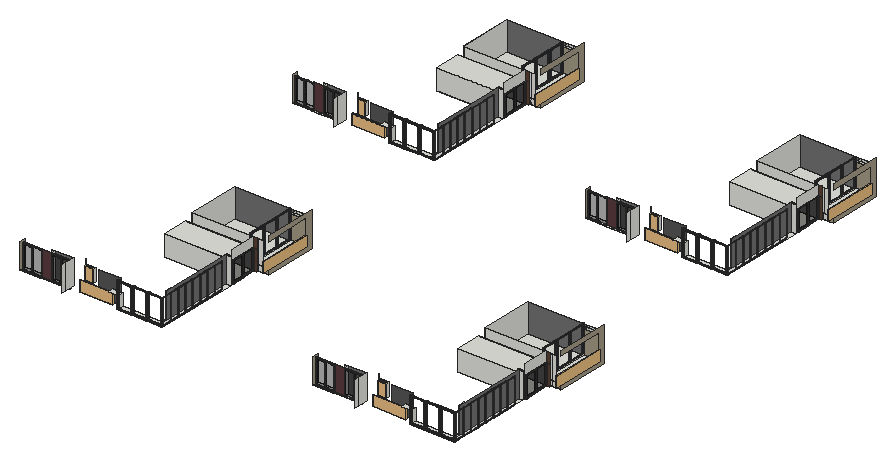
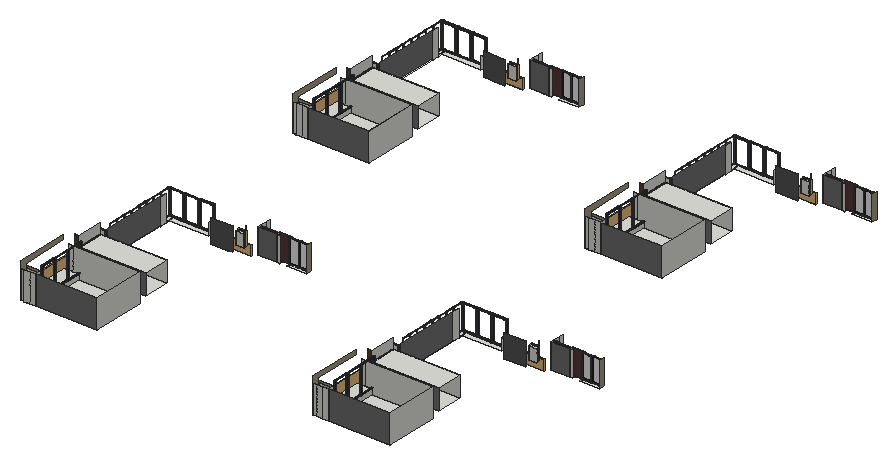
# SketchUp Ruby script. Lengths in inches.
U = 1.inch
M = Sketchup.active_model
def pt(a) = Geom::Point3d.new(a.map { |v| v * U })
def face(e, loops, mat)
  f = e.add_face(loops[0].map { |a| pt(a) })
  loops[1..].each { |l| e.add_face(l.map { |a| pt(a) }).erase! }
  f.material = f.back_material = mat if mat
  f
end
# faces: each face lists its corners as indices into pts; further lists are holes
def faces(e, pts, list, mat = nil) = list.each { |f| face(e, (f[0].is_a?(Array) ? f : [f]).map { |l| l.map { |i| pts[i] } }, mat) }
# xy, xz, yz: faces in a plane at the given z, y or x. An outline is a flat list of corners, or four numbers for a rectangle; further outlines are holes
def ring(l) = l.size == 4 ? [[l[0], l[1]], [l[2], l[1]], [l[2], l[3]], [l[0], l[3]]] : l.each_slice(2).to_a
def flat(e, list, mat, &to3) = list.each { |f| face(e, (f[0].is_a?(Array) ? f : [f]).map { |l| ring(l).map { |u, v| to3.(u, v) } }, mat) }
def xy(e, z, list, mat = nil) = flat(e, list, mat) { |x, y| [x, y, z] }
def xz(e, y, list, mat = nil) = flat(e, list, mat) { |x, z| [x, y, z] }
def yz(e, x, list, mat = nil) = flat(e, list, mat) { |y, z| [x, y, z] }
def lines(e, pts, list) = list.each { |a, b| e.add_line(pt(pts[a]), pt(pts[b])) }
# prism: a flat outline (further loops are holes) pulled along v
def prism(e, loops, v, mat = nil)
  f = face(e, loops, mat); d = Geom::Vector3d.new(v.map { |x| x * U })
  f.pushpull(f.normal.samedirection?(d) ? d.length : -d.length)
end
def box(e, o, s, mat = nil) = prism(e, [[o, [o[0] + s[0], o[1], o[2]], [o[0] + s[0], o[1] + s[1], o[2]], [o[0], o[1] + s[1], o[2]]]], [0, 0, s[2]], mat)
def at(x, y, z, deg = 0) = Geom::Transformation.translation(pt([x, y, z])) * Geom::Transformation.rotation(ORIGIN, Z_AXIS, deg.degrees)
def axes(o, x, y, z) = Geom::Transformation.new([*x, 0, *y, 0, *z, 0, *pt(o).to_a, 1])
def part(name) = M.definitions.add(name)
# library, detail: a bought-in or finely detailed component or shape, given as its bounding box
def library(name, o, s) = part(name).tap { |d| box(d.entities, o, s) }
def detail(e, o, s) = box(e.add_group.entities, o, s)
def put(e, d, t, mat = nil) = e.add_instance(d, t).tap { |i| i.material = mat if mat }
def group(e, t, mat = nil) = e.add_group.tap { |g| g.transformation = t; g.material = mat if mat }.entities
root = M.entities
M.materials.add("Glass_Tinted_Gray").color = [0, 0, 0]
M.materials["Glass_Tinted_Gray"].alpha = 0.125
M.materials.add("Glazing").color = [128, 128, 128]
M.materials["Glazing"].alpha = 0.05
M.materials.add("Powdercoating").color = [41, 44, 40]
M.materials.add("Wine2").color = [0, 0, 0]
M.materials["Wine2"].alpha = 0
M.materials.add("[0130_Gainsboro]").color = [39, 45, 50]
M.materials.add("[0135_DarkGray]").color = [81, 81, 81]
M.materials.add("[Color M05]").color = [114, 114, 114]
M.materials.add("[Color M06]").color = [86, 86, 86]
M.materials.add("[Concrete Tile]").color = [165, 155, 133]
M.materials.add("[Granite Brown]").color = [89, 59, 61]
M.materials.add("[Granite Brown]1").color = [89, 63, 50]
M.materials.add("[Mirror 02]").color = [229, 229, 229]
M.materials.add("[Terrazzo Light Blue]").color = [196, 214, 227]
c1 = library("Glass Railing",[0,0,0],[139.5,4.76,42])
c2 = part("PENTEK_RP Fineline 50S_Sliding_DoorCase_E1")
box(c2.entities,[0,0,0],[1.51,3.66,99.27],"[0135_DarkGray]")
c3 = part("PENTEK_RP Fineline 50S_SlidingDooe_Case_E2")
box(c3.entities,[0,0,0],[96.25,3.66,1.51],"[0135_DarkGray]")
c4 = part("pentek_RP Fineline 50S_SlidingDoor_Case")
put(c4.entities,c2,at(97.76,0,0))
put(c4.entities,c3,at(1.51,0,0))
put(c4.entities,c2,at(0,0,0))
put(c4.entities,c3,at(1.51,0,97.76))
c5 = part("PENTEK_RP Fineline 50S_SlidingDoor_GlazingBead_2")
box(c5.entities,[0,0,0],[0.56,0.59,94.39],"[0135_DarkGray]")
c6 = part("PENTEK_RP Fineline 50S_SlidingDoor_Glass")
box(c6.entities,[0,0,0],[46.58,0.16,94.39],"Glass_Tinted_Gray")
c7 = part("PENTEK_RP Fineline 50S_SlidingDoor_GlazingBead")
box(c7.entities,[0,0,0],[45.47,0.59,0.56],"[0135_DarkGray]")
c8 = part("PENTEK_RP Fineline 50S_SlidingDoor_Leaf_E1")
xy(c8.entities,0,[[0,0,0.93,1.97],[0.93,1.57,1.49,1.97]],"[0135_DarkGray]")
xy(c8.entities,96.25,[[0,0,0.93,0,0.93,1.57,1.49,1.57,1.49,1.97,0,1.97]],"[0135_DarkGray]")
xz(c8.entities,0,[[0,0,0.93,96.25]],"[0135_DarkGray]")
xz(c8.entities,1.57,[[0.93,0,1.49,95.32],[0.93,95.32,1.49,96.25]],"[0135_DarkGray]")
xz(c8.entities,1.97,[[0,0,1.49,96.25]],"[0135_DarkGray]")
yz(c8.entities,0,[[0,0,1.97,96.25]],"[0135_DarkGray]")
yz(c8.entities,0.93,[[0,0,1.57,0.93],[0,0.93,1.57,95.32],[0,95.32,1.57,96.25]],"[0135_DarkGray]")
yz(c8.entities,1.49,[[1.57,0,1.97,95.32],[1.57,95.32,1.97,96.25]],"[0135_DarkGray]")
c9 = part("PENTEK_RP Fineline 50S_SlidingDoor_Leaf_E2")
xy(c9.entities,0,[[0,0,0,1.57,0.56,1.57,0.56,1.97,46.02,1.97,46.02,1.57,46.58,1.57,46.58,0]],"[0135_DarkGray]")
xy(c9.entities,0.93,[[0,0,46.58,1.57]],"[0135_DarkGray]")
xy(c9.entities,1.49,[[0.56,1.57,46.02,1.97]],"[0135_DarkGray]")
xz(c9.entities,0,[[0,0,46.58,0.93]],"[0135_DarkGray]")
xz(c9.entities,1.57,[[0,0,0.56,0.93],[46.02,0,46.58,0.93],[0.56,0.93,46.02,1.49]],"[0135_DarkGray]")
xz(c9.entities,1.97,[[0.56,0,46.02,1.49]],"[0135_DarkGray]")
yz(c9.entities,0,[[0,0,1.57,0.93]],"[0135_DarkGray]")
yz(c9.entities,0.56,[[1.57,0,1.97,0.93],[1.57,0.93,1.97,1.49]],"[0135_DarkGray]")
yz(c9.entities,46.02,[[1.57,0,1.97,0.93],[1.57,0.93,1.97,1.49]],"[0135_DarkGray]")
yz(c9.entities,46.58,[[0,0,1.57,0.93]],"[0135_DarkGray]")
c10 = part("PENTEK_RP Fineline S_SlidingDoor_Leaf1")
put(c10.entities,c5,at(0.93,0,0.93))
put(c10.entities,c5,at(46.96,0,0.93))
put(c10.entities,c6,at(1.49,1.42,0.93))
put(c10.entities,c7,at(1.49,0,0.93))
put(c10.entities,c6,at(1.49,0.59,0.93),"[Terrazzo Light Blue]")
put(c10.entities,c8,at(0,0,0))
put(c10.entities,c8,axes([48.44,0,0],[-1,0,0],[0,1,0],[0,0,1]))
put(c10.entities,c9,axes([0.93,0,96.25],[1,0,0],[0,1,0],[0,0,-1]))
put(c10.entities,c9,at(0.93,0,0))
put(c10.entities,c7,at(1.49,0,94.77))
c11 = part("PENTEK_RP Fineline 50S_SlidingDoor_Leaf2")
put(c11.entities,c6,at(1.49,1.42,0.93))
put(c11.entities,c7,at(1.49,0,94.77))
put(c11.entities,c5,at(46.96,0,0.93))
put(c11.entities,c6,at(1.49,0.59,0.93),"[Mirror 02]")
put(c11.entities,c5,at(0.93,0,0.93))
put(c11.entities,c8,at(0,0,0))
put(c11.entities,c8,axes([48.44,0,0],[-1,0,0],[0,1,0],[0,0,1]))
put(c11.entities,c7,at(1.49,0,0.93))
put(c11.entities,c9,axes([0.93,0,96.25],[1,0,0],[0,1,0],[0,0,-1]))
put(c11.entities,c9,at(0.93,0,0))
c12 = part("PENTEK - Slimmest Steel Sliding Door / Window\#1")
put(c12.entities,c4,at(0,-1.88,-0.09))
put(c12.entities,c10,at(1.51,-2.27,1.42))
put(c12.entities,c11,at(49.32,-0.3,1.42))
c13 = part("Framed glazing panel")
xy(c13.entities,0,[[0,-0.98,43.07,0],[0,0,43.07,1.4]],"[0130_Gainsboro]")
xy(c13.entities,0.3,[[0.3,-1.43,42.77,-0.98]],"[0130_Gainsboro]")
xy(c13.entities,2.95,[[2.95,-1.43,40.12,-0.63],[2.95,-0.63,40.12,0],[2.95,0,40.12,0.64],[2.95,0.64,40.12,1.4]],"[0130_Gainsboro]")
xy(c13.entities,3.54,[[3.54,-0.63,39.53,0],[3.54,0,39.53,0.64]],"[0130_Gainsboro]")
xy(c13.entities,111.8125,[[3.54,-0.63,39.53,0],[3.54,0,39.53,0.64]],"[0130_Gainsboro]")
xy(c13.entities,112.4,[[2.95,-1.43,40.12,-0.63],[2.95,-0.63,40.12,0],[2.95,0,40.12,0.64],[2.95,0.64,40.12,1.4]],"[0130_Gainsboro]")
xy(c13.entities,115.05,[[0.3,-1.43,42.77,-0.98]],"[0130_Gainsboro]")
xy(c13.entities,115.35,[[0,-0.98,43.07,0],[0,0,43.07,1.4]],"[0130_Gainsboro]")
xz(c13.entities,-1.43,[[[0.3,0.3,42.77,115.05],[2.95,2.95,40.12,112.4]]],"[0130_Gainsboro]")
xz(c13.entities,-0.98,[[[0,0,43.07,115.35],[0.3,0.3,42.77,115.05]]],"[0130_Gainsboro]")
xz(c13.entities,-0.63,[[[2.95,2.95,40.12,112.4],[3.54,3.54,39.53,111.8125]]],"[0130_Gainsboro]")
xz(c13.entities,0,[[3.54,3.54,39.53,111.8125]],"Wine2")
xz(c13.entities,0,[[[0,0,43.07,115.35],[2.95,2.95,40.12,112.4]],[[2.95,2.95,40.12,112.4],[3.54,3.54,39.53,111.8125]]],"[0130_Gainsboro]")
xz(c13.entities,0.64,[[[2.95,2.95,40.12,112.4],[3.54,3.54,39.53,111.8125]]],"[0130_Gainsboro]")
xz(c13.entities,1.4,[[[0,0,43.07,115.35],[2.95,2.95,40.12,112.4]]],"[0130_Gainsboro]")
yz(c13.entities,0,[[-0.98,0,0,115.35],[0,0,1.4,115.35]],"[0130_Gainsboro]")
yz(c13.entities,0.3,[[-1.43,0.3,-0.98,115.05]],"[0130_Gainsboro]")
yz(c13.entities,2.95,[[-1.43,2.95,-0.63,112.4],[-0.63,2.95,0,112.4],[0,2.95,0.64,112.4],[0.64,2.95,1.4,112.4]],"[0130_Gainsboro]")
yz(c13.entities,3.54,[[-0.63,3.54,0,111.8125],[0,3.54,0.64,111.8125]],"[0130_Gainsboro]")
yz(c13.entities,39.53,[[-0.63,3.54,0,111.8125],[0,3.54,0.64,111.8125]],"[0130_Gainsboro]")
yz(c13.entities,40.12,[[-1.43,2.95,-0.63,112.4],[-0.63,2.95,0,112.4],[0,2.95,0.64,112.4],[0.64,2.95,1.4,112.4]],"[0130_Gainsboro]")
yz(c13.entities,42.77,[[-1.43,0.3,-0.98,115.05]],"[0130_Gainsboro]")
yz(c13.entities,43.07,[[-0.98,0,0,115.35],[0,0,1.4,115.35]],"[0130_Gainsboro]")
c14 = part("Glazed panel assembly")
put(c14.entities,c13,axes([90.57,1.43,0],[1.05148,0,0],[0,1,0],[0,0,1]))
put(c14.entities,c13,axes([0,1.43,0],[1.05148,0,0],[0,1,0],[0,0,1]))
put(c14.entities,c13,axes([45.29,1.43,0],[1.05148,0,0],[0,1,0],[0,0,1]))
c15 = part("Group\#15")
xy(c15.entities,0,[[0,-55.94,0.71,45.94]])
xy(c15.entities,0.2,[[0,-55.94,0.47,45.94],[0.47,45.94,0.71,46.42]])
xy(c15.entities,2.36,[[0.47,-55.94,0.71,46.42]])
xz(c15.entities,-55.94,[[0,0,0.71,0,0.71,2.36,0.47,2.36,0.47,0.2,0,0.2]])
xz(c15.entities,45.94,[[0,0,0.71,0.2]])
xz(c15.entities,46.42,[[0.47,0.2,0.71,2.36]])
yz(c15.entities,0,[[-55.94,0,45.94,0.2]])
yz(c15.entities,0.47,[[-55.94,0.2,46.42,2.36]])
yz(c15.entities,0.71,[[-55.94,0,45.94,0,45.94,0.2,46.42,0.2,46.42,2.36,-55.94,2.36]])
c16 = part("Group\#7")
xy(c16.entities,0,[[0,-59.09,0.71,45.94]])
xy(c16.entities,0.2,[[0,-59.09,0.47,45.94],[0.47,45.94,0.71,46.42]])
xy(c16.entities,2.36,[[0.47,-59.09,0.71,46.42]])
xz(c16.entities,-59.09,[[0,0,0.71,0,0.71,2.36,0.47,2.36,0.47,0.2,0,0.2]])
xz(c16.entities,45.94,[[0,0,0.71,0.2]])
xz(c16.entities,46.42,[[0.47,0.2,0.71,2.36]])
yz(c16.entities,0,[[-59.09,0,45.94,0.2]])
yz(c16.entities,0.47,[[-59.09,0.2,46.42,2.36]])
yz(c16.entities,0.71,[[-59.09,0,45.94,0,45.94,0.2,46.42,0.2,46.42,2.36,-59.09,2.36]])
c17 = part("Group\#16")
prism(c17.entities,[[[0.47,-56.18,0.2],[0,-56.18,0.2],[0,-56.18,0],[0.71,-56.18,0],[0.71,-56.18,2.36],[0.47,-56.18,2.36]]],[0,28.68,0])
c18 = part("Group\#10")
box(c18.entities,[-0.73,0,0],[27.99,0.55,102.05])
c19 = part("Group\#18")
xy(c19.entities,0,[[0.47,-56.18,0.47,-55.47,0,-55.47,0,-28.21,1.18,-28.21,1.18,-56.18]])
xy(c19.entities,0.2,[[0.71,-56.18,1.18,-28.21],[0,-55.47,0.47,-28.21],[0.47,-28.21,0.71,-27.74]])
xy(c19.entities,2.36,[[0.47,-56.18,0.71,-27.74]])
xz(c19.entities,-56.18,[[0.47,0,1.18,0,1.18,0.2,0.71,0.2,0.71,2.36,0.47,2.36]])
xz(c19.entities,-55.47,[[0,0,0.47,0.2]])
xz(c19.entities,-28.21,[[0,0,1.18,0.2]])
xz(c19.entities,-27.74,[[0.47,0.2,0.71,2.36]])
yz(c19.entities,0,[[-55.47,0,-28.21,0.2]])
yz(c19.entities,0.47,[[-56.18,0,-55.47,0.2],[-56.18,0.2,-27.74,2.36]])
yz(c19.entities,0.71,[[-56.18,0.2,-27.74,2.36]])
yz(c19.entities,1.18,[[-56.18,0,-28.21,0.2]])
c20 = part("Group\#34")
xy(c20.entities,0,[[-20.45,0,7.76,1.22]])
xy(c20.entities,0.06,[[-20.39,0.06,7.7,1.22]])
xy(c20.entities,0.47,[[-19.98,0,7.28,0.06]])
xy(c20.entities,101.89,[[-19.98,0,7.28,0.06]])
xy(c20.entities,102.3,[[-20.39,0.06,7.7,1.22]])
xy(c20.entities,102.36,[[-20.45,0,7.76,1.22]])
xz(c20.entities,0,[[[-20.45,0,7.76,102.36],[-19.98,0.47,7.28,101.89]]])
xz(c20.entities,0.06,[[[-20.39,0.06,7.7,102.3],[-19.98,0.47,7.28,101.89]]])
xz(c20.entities,1.22,[[[-20.45,0,7.76,102.36],[-20.39,0.06,7.7,102.3]]])
yz(c20.entities,-20.45,[[0,0,1.22,102.36]])
yz(c20.entities,-20.39,[[0.06,0.06,1.22,102.3]])
yz(c20.entities,-19.98,[[0,0.47,0.06,101.89]])
yz(c20.entities,7.28,[[0,0.47,0.06,101.89]])
yz(c20.entities,7.7,[[0.06,0.06,1.22,102.3]])
yz(c20.entities,7.76,[[0,0,1.22,102.36]])
c21 = part("Group\#6")
put(c21.entities,c15,axes([27.97,0,7.875],[1,0,0],[0,0,-1],[0,1,0]),"Powdercoating")
put(c21.entities,c16,axes([0.71,0,6.8],[-1,0,0],[0,0,-0.97687],[0,1,0]),"Powdercoating")
put(c21.entities,c17,axes([-27.5,0,-38.07],[0,0,-1],[-1,0,0],[0,1,0]),"Powdercoating")
put(c21.entities,c18,at(1.12,0.35,-38.39),"Glazing")
put(c21.entities,c19,axes([-27.5,0,63.35],[0,0,1],[-1,0,0],[0,1,0]),"Powdercoating")
put(c21.entities,c20,at(20.6875,1.0625,-38.54),"Powdercoating")
c22 = part("Sliding door assembly")
put(c22.entities,c21,at(-1.18,4.5,38.86))
g1 = group(c22.entities,at(84.74,4.5,38.86))
put(g1,c15,axes([-27.97,0,7.875],[-1,0,0],[0,0,-1],[0,1,0]),"Powdercoating")
put(g1,c16,axes([-0.71,0,6.8],[1,0,0],[0,0,-0.97687],[0,1,0]),"Powdercoating")
put(g1,c17,axes([27.5,0,-38.07],[0,0,-1],[1,0,0],[0,1,0]),"Powdercoating")
put(g1,c18,axes([-1.12,0.35,-38.39],[-1,0,0],[0,1,0],[0,0,1]),"Glazing")
put(g1,c19,axes([27.5,0,63.35],[0,0,1],[1,0,0],[0,1,0]),"Powdercoating")
put(g1,c20,axes([-20.6875,1.0625,-38.54],[-1,0,0],[0,1,0],[0,0,1]),"Powdercoating")
g2 = group(c22.entities,at(56.0625,4.5,38.86))
put(g2,c15,axes([-27.97,0,7.875],[-1,0,0],[0,0,-1],[0,1,0]),"Powdercoating")
put(g2,c17,axes([27.5,0,-38.07],[0,0,-1],[1,0,0],[0,1,0]),"Powdercoating")
put(g2,c18,axes([-1.12,0.35,-38.39],[-1,0,0],[0,1,0],[0,0,1]),"Glazing")
put(g2,c19,axes([27.5,0,63.35],[0,0,1],[1,0,0],[0,1,0]),"Powdercoating")
put(g2,c20,axes([-20.6875,1.0625,-38.54],[-1,0,0],[0,1,0],[0,0,1]),"Powdercoating")
g3 = group(g2,at(-0.71,0,6.8),"Powdercoating")
xy(g3,-45.34,[[0.47,0.2,0.71,2.36]])
xy(g3,-44.88,[[0,0,0.71,0.2]])
xy(g3,57.73,[[0,0,0.71,0,0.71,2.36,0.47,2.36,0.47,0.2,0,0.2]])
xz(g3,0,[[0,-44.88,0.71,57.73]])
xz(g3,0.2,[[0.47,-45.34,0.71,-44.88],[0,-44.88,0.47,57.73]])
xz(g3,2.36,[[0.47,-45.34,0.71,57.73]])
yz(g3,0,[[0,-44.88,0.2,57.73]])
yz(g3,0.47,[[0.2,-45.34,2.36,57.73]])
yz(g3,0.71,[[0.2,-45.34,2.36,-45.34,2.36,57.73,0,57.73,0,-44.88,0.2,-44.88]])
put(c22.entities,c21,axes([-33.94,4.5,38.86],[1.14218,0,0],[0,1,0],[0,0,1]))
c23 = part("sliding door")
put(c23.entities,c22,at(0,-4.5,-0.08))
c24 = library("Klein+raam",[128.36,12.7,0],[19.68,5.51,55.12])
xy(root,763.75,[[635.3125,2295.875,637.0625,2518.89],[637.0625,2295.875,889.625,2518.89],[889.625,2295.875,890.875,2518.89],[890.875,2295.875,938.375,2518.89],[938.375,2295.875,938.5625,2518.89],
  [938.5625,2295.875,954.6875,2518.89],[1853.5,2295.875,1855.25,2518.89],[1855.25,2295.875,2107.8125,2518.89],[2107.8125,2295.875,2109.0625,2518.89],[2109.0625,2295.875,2156.5625,2518.89],
  [2156.5625,2295.875,2156.75,2518.89],[2156.75,2295.875,2172.875,2518.89],[635.3125,3710.5625,637.0625,3933.57],[637.0625,3710.5625,889.625,3933.57],[889.625,3710.5625,890.875,3933.57],
  [890.875,3710.5625,938.375,3933.57],[938.375,3710.5625,938.5625,3933.57],[938.5625,3710.5625,954.6875,3933.57],[1853.5,3710.5625,1855.25,3933.57],[1855.25,3710.5625,2107.8125,3933.57],
  [2107.8125,3710.5625,2109.0625,3933.57],[2109.0625,3710.5625,2156.5625,3933.57],[2156.5625,3710.5625,2156.75,3933.57],[2156.75,3710.5625,2172.875,3933.57]])
xy(root,774.75,[[727.43,1799.9375,890.875,1822.9375],[890.875,1799.9375,891.6875,1842.5],[891.6875,1799.9375,894,1842.5],[894,1799.9375,894.3125,1842.5],[894.3125,1799.9375,913.875,2148.83],
  [1945.62,1799.9375,2109.0625,1822.9375],[2109.0625,1799.9375,2109.875,1842.5],[2109.875,1799.9375,2112.1875,1842.5],[2112.1875,1799.9375,2112.5,1842.5],[2112.5,1799.9375,2132.0625,2148.83],
  [890.875,1842.5,891.6875,1869.5],[891.6875,1842.5,894,2148.83],[894,1842.5,894.3125,2148.83],[2109.0625,1842.5,2109.875,1869.5],[2109.875,1842.5,2112.1875,2148.83],
  [2112.1875,1842.5,2112.5,2148.83],[727.43,3214.625,890.875,3237.625],[890.875,3214.625,891.6875,3257.1875],[891.6875,3214.625,894,3257.1875],[894,3214.625,894.3125,3257.1875],
  [894.3125,3214.625,913.875,3563.51],[1945.62,3214.625,2109.0625,3237.625],[2109.0625,3214.625,2109.875,3257.1875],[2109.875,3214.625,2112.1875,3257.1875],[2112.1875,3214.625,2112.5,3257.1875],
  [2112.5,3214.625,2132.0625,3563.51],[890.875,3257.1875,891.6875,3284.1875],[891.6875,3257.1875,894,3563.51],[894,3257.1875,894.3125,3563.51],[2109.0625,3257.1875,2109.875,3284.1875],
  [2109.875,3257.1875,2112.1875,3563.51],[2112.1875,3257.1875,2112.5,3563.51]])
xy(root,777.4375,[[319.53,1799.9375,402.43,1822.9375],[402.43,1799.9375,431.33,1806.5625],[431.33,1799.9375,523.04,1799.9375,523.04,1822.9375,446.15,1822.9375,446.15,1806.5625,431.33,1806.5625],[1537.72,1799.9375,1620.62,1822.9375],[1620.62,1799.9375,1649.52,1806.5625],
  [1649.52,1799.9375,1741.23,1799.9375,1741.23,1822.9375,1664.33,1822.9375,1664.33,1806.5625,1649.52,1806.5625],[431.33,1806.5625,446.15,1822.9375],[1649.52,1806.5625,1664.33,1822.9375],[319.53,3214.625,402.43,3237.625],[402.43,3214.625,431.33,3221.25],
  [431.33,3214.625,523.04,3214.625,523.04,3237.625,446.15,3237.625,446.15,3221.25,431.33,3221.25],[1537.72,3214.625,1620.62,3237.625],[1620.62,3214.625,1649.52,3221.25],[1649.52,3214.625,1741.23,3214.625,1741.23,3237.625,1664.33,3237.625,1664.33,3221.25,1649.52,3221.25],[431.33,3221.25,446.15,3237.625],
  [1649.52,3221.25,1664.33,3237.625]])
xy(root,779.36,[[635.3125,2156.01,913.875,2266.33],[1853.5,2156.01,2132.0625,2266.33],[635.3125,3570.7,913.875,3681.01],[1853.5,3570.7,2132.0625,3681.01]])
xy(root,786.0625,[[889.625,2295.875,890.875,2492.875],[890.875,2295.875,954.6875,2492.875],[2107.8125,2295.875,2109.0625,2492.875],[2109.0625,2295.875,2172.875,2492.875],[890.875,2492.875,938.375,2505.5625],
  [2109.0625,2492.875,2156.5625,2505.5625],[889.625,3710.5625,890.875,3907.5625],[890.875,3710.5625,954.6875,3907.5625],[2107.8125,3710.5625,2109.0625,3907.5625],[2109.0625,3710.5625,2172.875,3907.5625],
  [890.875,3907.5625,938.375,3920.25],[2109.0625,3907.5625,2156.5625,3920.25]])
xy(root,805.12,[[557.88,1842.5,589.71,1853.125],[1776.07,1842.5,1807.9,1853.125],[557.88,3257.1875,589.71,3267.8125],[1776.07,3257.1875,1807.9,3267.8125]])
xy(root,805.12,[[557.4,1842.5,557.88,1853.125],[1775.59,1842.5,1776.07,1853.125],[557.4,3257.1875,557.88,3267.8125],[1775.59,3257.1875,1776.07,3267.8125]],"[Granite Brown]")
xy(root,825,[[686.18,1799.9375,727.43,1822.9375],[1904.37,1799.9375,1945.62,1822.9375],[686.18,3214.625,727.43,3237.625],[1904.37,3214.625,1945.62,3237.625]])
xy(root,857.4,[[557.88,1842.5,589.71,1853.125],[1776.07,1842.5,1807.9,1853.125],[557.88,3257.1875,589.71,3267.8125],[1776.07,3257.1875,1807.9,3267.8125]])
xy(root,857.4,[[557.4,1842.5,557.88,1853.125],[1775.59,1842.5,1776.07,1853.125],[557.4,3257.1875,557.88,3267.8125],[1775.59,3257.1875,1776.07,3267.8125]],"[Granite Brown]")
xy(root,865.04,[[635.3125,2156.01,913.875,2266.33],[1853.5,2156.01,2132.0625,2266.33],[635.3125,3570.7,913.875,3681.01],[1853.5,3570.7,2132.0625,3681.01]])
xz(root,1806.5625,[[402.51,777.4375,446.15,777.4375,446.15,882,403.03,882],[1620.7,777.4375,1664.33,777.4375,1664.33,882,1621.22,882]],"[Granite Brown]")
xz(root,1822.9375,[[431.33,777.4375,446.15,882],[1649.52,777.4375,1664.33,882]])
xz(root,1822.9375,[[446.15,777.4375,523.04,882],[1664.33,777.4375,1741.23,882]],"[Color M05]")
xz(root,1842.5,[[891.6875,774.75,894.3125,882],[2109.875,774.75,2112.5,882]])
xz(root,1842.5,[[632.49,763.875,701.59,763.875,701.59,862,611.65,862,611.65,764.1875,632.49,764.1875],[1850.67,763.875,1919.77,763.875,1919.77,862,1829.84,862,1829.84,764.1875,1850.67,764.1875]],"[Color M06]")
xz(root,1842.5,[[557.4,857.4,557.88,882],[1775.59,857.4,1776.07,882]],"[Granite Brown]")
xz(root,1853.125,[[557.88,805.12,589.71,857.4],[1776.07,805.12,1807.9,857.4]])
xz(root,1853.125,[[557.4,805.12,557.88,857.4],[1775.59,805.12,1776.07,857.4]],"[Granite Brown]")
xz(root,2148.83,[[891.6875,774.75,894,882],[894,774.75,894.3125,882],[894.3125,774.75,913.875,882],[2109.875,774.75,2112.1875,882],[2112.1875,774.75,2112.5,882],
  [2112.5,774.75,2132.0625,882]])
xz(root,2156.01,[[635.3125,779.36,894,865.04],[894,779.36,894.3125,865.04],[894.3125,779.36,913.875,865.04],[1853.5,779.36,2112.1875,865.04],[2112.1875,779.36,2112.5,865.04],
  [2112.5,779.36,2132.0625,865.04],[894,865.04,894.3125,882],[894.3125,865.04,913.875,882],[2112.1875,865.04,2112.5,882],[2112.5,865.04,2132.0625,882]])
xz(root,2266.33,[[635.3125,779.36,913.875,865.04],[1853.5,779.36,2132.0625,865.04]],"[Color M05]")
xz(root,2266.33,[[913.875,779.36,930.75,865.04],[2132.0625,779.36,2148.9375,865.04],[913.875,865.04,930.75,905.36],[2132.0625,865.04,2148.9375,905.36]],"[Granite Brown]1")
xz(root,2295.875,[[635.3125,763.75,637.0625,882],[637.0625,763.75,637.0625,882,913.875,882,913.875,786.0625,889.625,786.0625,889.625,763.75],[889.625,763.75,890.875,786.0625],[890.875,763.75,913.875,786.0625],[913.875,763.75,930.75,786.0625],
  [938.375,763.75,938.5625,786.0625],[1853.5,763.75,1855.25,882],[1855.25,763.75,1855.25,882,2132.0625,882,2132.0625,786.0625,2107.8125,786.0625,2107.8125,763.75],[2107.8125,763.75,2109.0625,786.0625],[2109.0625,763.75,2132.0625,786.0625],
  [2132.0625,763.75,2148.9375,786.0625],[2156.5625,763.75,2156.75,786.0625],[913.875,786.0625,930.75,882],[2132.0625,786.0625,2148.9375,882]])
xz(root,2295.875,[[930.75,763.75,938.375,786.0625],[938.5625,763.75,954.6875,786.0625],[2148.9375,763.75,2156.5625,786.0625],[2156.75,763.75,2172.875,786.0625]],"[Concrete Tile]")
xz(root,2492.875,[[889.625,786.0625,954.6875,882],[2107.8125,786.0625,2172.875,882]],"[Concrete Tile]")
xz(root,2505.5625,[[890.875,786.0625,938.375,882],[2109.0625,786.0625,2156.5625,882]])
xz(root,2518.89,[[635.3125,763.75,637.0625,882],[889.625,763.75,890.875,882],[890.875,763.75,913.875,882],[913.875,763.75,938.375,882],[938.375,763.75,938.5625,882],
  [938.5625,763.75,954.6875,882],[1853.5,763.75,1855.25,882],[2107.8125,763.75,2109.0625,882],[2109.0625,763.75,2132.0625,882],[2132.0625,763.75,2156.5625,882],
  [2156.5625,763.75,2156.75,882],[2156.75,763.75,2172.875,882]])
xz(root,2518.89,[[637.0625,763.75,889.625,882],[1855.25,763.75,2107.8125,882]],"[Color M05]")
xz(root,3221.25,[[402.51,777.4375,446.15,777.4375,446.15,882,403.03,882],[1620.7,777.4375,1664.33,777.4375,1664.33,882,1621.22,882]],"[Granite Brown]")
xz(root,3237.625,[[431.33,777.4375,446.15,882],[1649.52,777.4375,1664.33,882]])
xz(root,3237.625,[[446.15,777.4375,523.04,882],[1664.33,777.4375,1741.23,882]],"[Color M05]")
xz(root,3257.1875,[[891.6875,774.75,894.3125,882],[2109.875,774.75,2112.5,882]])
xz(root,3257.1875,[[632.49,763.875,701.59,763.875,701.59,862,611.65,862,611.65,764.1875,632.49,764.1875],[1850.67,763.875,1919.77,763.875,1919.77,862,1829.84,862,1829.84,764.1875,1850.67,764.1875]],"[Color M06]")
xz(root,3257.1875,[[557.4,857.4,557.88,882],[1775.59,857.4,1776.07,882]],"[Granite Brown]")
xz(root,3267.8125,[[557.88,805.12,589.71,857.4],[1776.07,805.12,1807.9,857.4]])
xz(root,3267.8125,[[557.4,805.12,557.88,857.4],[1775.59,805.12,1776.07,857.4]],"[Granite Brown]")
xz(root,3563.51,[[891.6875,774.75,894,882],[894,774.75,894.3125,882],[894.3125,774.75,913.875,882],[2109.875,774.75,2112.1875,882],[2112.1875,774.75,2112.5,882],
  [2112.5,774.75,2132.0625,882]])
xz(root,3570.7,[[635.3125,779.36,894,865.04],[894,779.36,894.3125,865.04],[894.3125,779.36,913.875,865.04],[1853.5,779.36,2112.1875,865.04],[2112.1875,779.36,2112.5,865.04],
  [2112.5,779.36,2132.0625,865.04],[894,865.04,894.3125,882],[894.3125,865.04,913.875,882],[2112.1875,865.04,2112.5,882],[2112.5,865.04,2132.0625,882]])
xz(root,3681.01,[[635.3125,779.36,913.875,865.04],[1853.5,779.36,2132.0625,865.04]],"[Color M05]")
xz(root,3681.01,[[913.875,779.36,930.75,865.04],[2132.0625,779.36,2148.9375,865.04],[913.875,865.04,930.75,905.36],[2132.0625,865.04,2148.9375,905.36]],"[Granite Brown]1")
xz(root,3710.5625,[[635.3125,763.75,637.0625,882],[637.0625,763.75,637.0625,882,913.875,882,913.875,786.0625,889.625,786.0625,889.625,763.75],[889.625,763.75,890.875,786.0625],[890.875,763.75,913.875,786.0625],[913.875,763.75,930.75,786.0625],
  [938.375,763.75,938.5625,786.0625],[1853.5,763.75,1855.25,882],[1855.25,763.75,1855.25,882,2132.0625,882,2132.0625,786.0625,2107.8125,786.0625,2107.8125,763.75],[2107.8125,763.75,2109.0625,786.0625],[2109.0625,763.75,2132.0625,786.0625],
  [2132.0625,763.75,2148.9375,786.0625],[2156.5625,763.75,2156.75,786.0625],[913.875,786.0625,930.75,882],[2132.0625,786.0625,2148.9375,882]])
xz(root,3710.5625,[[930.75,763.75,938.375,786.0625],[938.5625,763.75,954.6875,786.0625],[2148.9375,763.75,2156.5625,786.0625],[2156.75,763.75,2172.875,786.0625]],"[Concrete Tile]")
xz(root,3907.5625,[[889.625,786.0625,954.6875,882],[2107.8125,786.0625,2172.875,882]],"[Concrete Tile]")
xz(root,3920.25,[[890.875,786.0625,938.375,882],[2109.0625,786.0625,2156.5625,882]])
xz(root,3933.57,[[635.3125,763.75,637.0625,882],[889.625,763.75,890.875,882],[890.875,763.75,913.875,882],[913.875,763.75,938.375,882],[938.375,763.75,938.5625,882],
  [938.5625,763.75,954.6875,882],[1853.5,763.75,1855.25,882],[2107.8125,763.75,2109.0625,882],[2109.0625,763.75,2132.0625,882],[2132.0625,763.75,2156.5625,882],
  [2156.5625,763.75,2156.75,882],[2156.75,763.75,2172.875,882]])
xz(root,3933.57,[[637.0625,763.75,889.625,882],[1855.25,763.75,2107.8125,882]],"[Color M05]")
yz(root,319.53,[[1799.9375,777.4375,1822.9375,882],[3214.625,777.4375,3237.625,882]],"[Concrete Tile]")
yz(root,446.15,[[1806.5625,777.4375,1822.9375,882],[3221.25,777.4375,3237.625,882]])
yz(root,523.04,[[1763.25,777.4375,1822.9375,882],[3177.9375,777.4375,3237.625,882]])
yz(root,589.71,[[1842.5,805.12,1853.125,857.4],[3257.1875,805.12,3267.8125,857.4]])
yz(root,635.3125,[[2295.875,763.75,2518.89,882],[3710.5625,763.75,3933.57,882]])
yz(root,637.0625,[[2295.875,763.75,2518.89,882],[3710.5625,763.75,3933.57,882]])
yz(root,727.43,[[1799.9375,774.75,1822.9375,825],[3214.625,774.75,3237.625,825]])
yz(root,889.625,[[2295.875,763.75,2295.875,786.0625,2492.875,786.0625,2492.875,882,2518.89,882,2518.89,763.75],[3710.5625,763.75,3710.5625,786.0625,3907.5625,786.0625,3907.5625,882,3933.57,882,3933.57,763.75]])
yz(root,890.875,[[2295.875,763.75,2295.875,786.0625,2505.5625,786.0625,2505.5625,882,2518.89,882,2518.89,763.75],[3710.5625,763.75,3710.5625,786.0625,3920.25,786.0625,3920.25,882,3933.57,882,3933.57,763.75]])
yz(root,891.6875,[[1842.5,774.75,1869.5,882],[3257.1875,774.75,3284.1875,882]])
yz(root,894.3125,[[1842.5,774.75,2148.83,882],[3257.1875,774.75,3563.51,882]],"[Color M05]")
yz(root,913.875,[[2156.01,865.04,2266.33,905.36],[3570.7,865.04,3681.01,905.36]])
yz(root,954.6875,[[2295.875,763.75,2518.89,763.75,2518.89,908.8125,2295.875,908.8125,2295.875,888,2492.875,888,2492.875,786.0625,2295.875,786.0625],[3710.5625,763.75,3933.57,763.75,3933.57,908.8125,3710.5625,908.8125,3710.5625,888,3907.5625,888,3907.5625,786.0625,3710.5625,786.0625]],"[Concrete Tile]")
yz(root,1537.72,[[1799.9375,777.4375,1822.9375,882],[3214.625,777.4375,3237.625,882]],"[Concrete Tile]")
yz(root,1664.33,[[1806.5625,777.4375,1822.9375,882],[3221.25,777.4375,3237.625,882]])
yz(root,1741.23,[[1763.25,777.4375,1822.9375,882],[3177.9375,777.4375,3237.625,882]])
yz(root,1807.9,[[1842.5,805.12,1853.125,857.4],[3257.1875,805.12,3267.8125,857.4]])
yz(root,1853.5,[[2295.875,763.75,2518.89,882],[3710.5625,763.75,3933.57,882]])
yz(root,1855.25,[[2295.875,763.75,2518.89,882],[3710.5625,763.75,3933.57,882]])
yz(root,1945.62,[[1799.9375,774.75,1822.9375,825],[3214.625,774.75,3237.625,825]])
yz(root,2107.8125,[[2295.875,763.75,2295.875,786.0625,2492.875,786.0625,2492.875,882,2518.89,882,2518.89,763.75],[3710.5625,763.75,3710.5625,786.0625,3907.5625,786.0625,3907.5625,882,3933.57,882,3933.57,763.75]])
yz(root,2109.0625,[[2295.875,763.75,2295.875,786.0625,2505.5625,786.0625,2505.5625,882,2518.89,882,2518.89,763.75],[3710.5625,763.75,3710.5625,786.0625,3920.25,786.0625,3920.25,882,3933.57,882,3933.57,763.75]])
yz(root,2109.875,[[1842.5,774.75,1869.5,882],[3257.1875,774.75,3284.1875,882]])
yz(root,2112.5,[[1842.5,774.75,2148.83,882],[3257.1875,774.75,3563.51,882]],"[Color M05]")
yz(root,2132.0625,[[2156.01,865.04,2266.33,905.36],[3570.7,865.04,3681.01,905.36]])
yz(root,2172.875,[[2295.875,763.75,2518.89,763.75,2518.89,908.8125,2295.875,908.8125,2295.875,888,2492.875,888,2492.875,786.0625,2295.875,786.0625],[3710.5625,763.75,3933.57,763.75,3933.57,908.8125,3710.5625,908.8125,3710.5625,888,3907.5625,888,3907.5625,786.0625,3710.5625,786.0625]],"[Concrete Tile]")
p = [[1741.23,1778.3125,777.4375],[1741.23,1778.3125,882],[523.04,1778.3125,777.4375],[523.04,1778.3125,882],[1741.23,3193,777.4375],[1741.23,3193,882],
  [523.04,3193,777.4375],[523.04,3193,882]]
lines(root,p,[[0,1],[2,3],[4,5],[6,7]])
put(root,c1,at(1764.87,1823.74,765.97))
put(root,c1,at(546.68,1823.74,765.97))
put(root,c1,at(1764.87,3238.43,765.97))
put(root,c1,at(546.68,3238.43,765.97))
put(root,c12,axes([1662,1808.5625,774.375],[0.77709,0,0],[0,0.88,0],[0,0,1.054]))
put(root,c12,axes([443.82,1808.5625,774.375],[0.77709,0,0],[0,0.88,0],[0,0,1.054]))
put(root,c12,axes([1662,3223.25,774.375],[0.77709,0,0],[0,0.88,0],[0,0,1.054]))
put(root,c12,axes([443.82,3223.25,774.375],[0.77709,0,0],[0,0.88,0],[0,0,1.054]))
put(root,c14,axes([1943.5,1795.6875,774.75],[1.38,0,0],[0,1.50139,0],[0,0,0.93798]))
put(root,c14,axes([725.3125,1795.6875,774.75],[1.38,0,0],[0,1.50139,0],[0,0,0.93798]))
put(root,c14,axes([1943.5,3210.375,774.75],[1.38,0,0],[0,1.50139,0],[0,0,0.93798]))
put(root,c14,axes([725.3125,3210.375,774.75],[1.38,0,0],[0,1.50139,0],[0,0,0.93798]))
put(root,c23,axes([2131.2,1997.35,774.75],[0,1.302,0],[-1,0,0],[0,0,1.03877]))
put(root,c23,axes([2131.2,1843.2,774.75],[0,1.302,0],[-1,0,0],[0,0,1.03877]))
put(root,c23,axes([913.01,1997.35,774.75],[0,1.302,0],[-1,0,0],[0,0,1.03877]))
put(root,c23,axes([913.01,1843.2,774.75],[0,1.302,0],[-1,0,0],[0,0,1.03877]))
put(root,c23,axes([2131.2,3257.89,774.75],[0,1.302,0],[-1,0,0],[0,0,1.03877]))
put(root,c23,axes([2131.2,3412.03,774.75],[0,1.302,0],[-1,0,0],[0,0,1.03877]))
put(root,c23,axes([913.01,3412.03,774.75],[0,1.302,0],[-1,0,0],[0,0,1.03877]))
put(root,c23,axes([913.01,3257.89,774.75],[0,1.302,0],[-1,0,0],[0,0,1.03877]))
put(root,c12,axes([1545.375,1806.83,774.96],[0.77709,0,0],[0,0.88,0],[0,0,1.054]),"[Concrete Tile]")
put(root,c12,axes([327.1875,1806.83,774.96],[0.77709,0,0],[0,0.88,0],[0,0,1.054]),"[Concrete Tile]")
put(root,c12,axes([1545.375,3221.52,774.96],[0.77709,0,0],[0,0.88,0],[0,0,1.054]),"[Concrete Tile]")
put(root,c12,axes([327.1875,3221.52,774.96],[0.77709,0,0],[0,0.88,0],[0,0,1.054]),"[Concrete Tile]")
put(root,c12,axes([2131.3,2158.32,776.8],[0,1.12181,0],[-2.51374,0,0],[0,0,0.87918]))
put(root,c12,axes([913.11,2158.32,776.8],[0,1.12181,0],[-2.51374,0,0],[0,0,0.87918]))
put(root,c12,axes([2131.3,3573.01,776.8],[0,1.12181,0],[-2.51374,0,0],[0,0,0.87918]))
put(root,c12,axes([913.11,3573.01,776.8],[0,1.12181,0],[-2.51374,0,0],[0,0,0.87918]))
put(root,c1,axes([2174.63,2269.68,782.49],[0,1.6,0],[-1,0,0],[0,0,1]))
put(root,c1,axes([956.45,2269.68,782.49],[0,1.6,0],[-1,0,0],[0,0,1]))
put(root,c1,axes([2174.63,3684.36,782.49],[0,1.6,0],[-1,0,0],[0,0,1]))
put(root,c1,axes([956.45,3684.36,782.49],[0,1.6,0],[-1,0,0],[0,0,1]))
put(root,c14,axes([2108.26,2283.54,786.0625],[0,1.54079,0],[-1,0,0],[0,0,1]))
put(root,c14,axes([890.08,2283.54,786.0625],[0,1.54079,0],[-1,0,0],[0,0,1]))
put(root,c14,axes([2108.26,3698.23,786.0625],[0,1.54079,0],[-1,0,0],[0,0,1]))
put(root,c14,axes([890.08,3698.23,786.0625],[0,1.54079,0],[-1,0,0],[0,0,1]))
put(root,c24,axes([1572.84,1830.12,805.12],[1.58777,0,0],[0,0.68,0],[0,0,0.99202]))
put(root,c24,axes([354.65,1830.12,805.12],[1.58777,0,0],[0,0.68,0],[0,0,0.99202]))
put(root,c24,axes([1572.84,3244.81,805.12],[1.58777,0,0],[0,0.68,0],[0,0,0.99202]))
put(root,c24,axes([354.65,3244.81,805.12],[1.58777,0,0],[0,0.68,0],[0,0,0.99202]))
